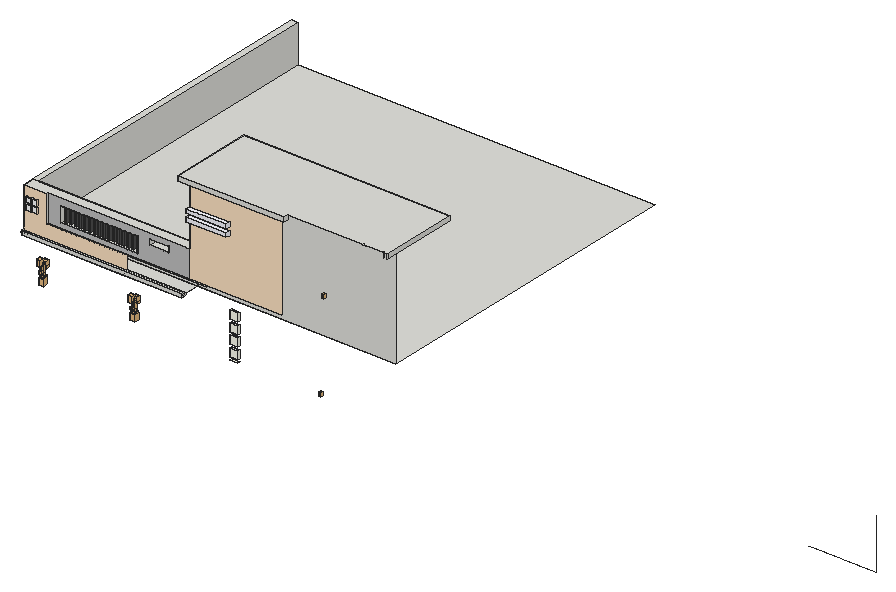
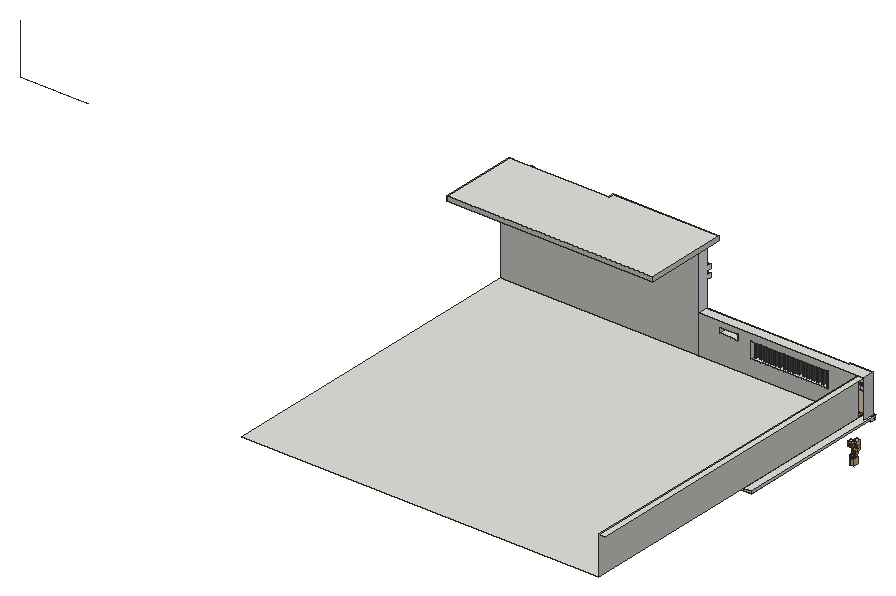
# SketchUp Ruby script. Lengths in inches.
U = 1.inch
M = Sketchup.active_model
def pt(a) = Geom::Point3d.new(a.map { |v| v * U })
def face(e, loops, mat)
  f = e.add_face(loops[0].map { |a| pt(a) })
  loops[1..].each { |l| e.add_face(l.map { |a| pt(a) }).erase! }
  f.material = f.back_material = mat if mat
  f
end
# faces: each face lists its corners as indices into pts; further lists are holes
def faces(e, pts, list, mat = nil) = list.each { |f| face(e, (f[0].is_a?(Array) ? f : [f]).map { |l| l.map { |i| pts[i] } }, mat) }
# xy, xz, yz: faces in a plane at the given z, y or x. An outline is a flat list of corners, or four numbers for a rectangle; further outlines are holes
def ring(l) = l.size == 4 ? [[l[0], l[1]], [l[2], l[1]], [l[2], l[3]], [l[0], l[3]]] : l.each_slice(2).to_a
def flat(e, list, mat, &to3) = list.each { |f| face(e, (f[0].is_a?(Array) ? f : [f]).map { |l| ring(l).map { |u, v| to3.(u, v) } }, mat) }
def xy(e, z, list, mat = nil) = flat(e, list, mat) { |x, y| [x, y, z] }
def xz(e, y, list, mat = nil) = flat(e, list, mat) { |x, z| [x, y, z] }
def yz(e, x, list, mat = nil) = flat(e, list, mat) { |y, z| [x, y, z] }
def lines(e, pts, list) = list.each { |a, b| e.add_line(pt(pts[a]), pt(pts[b])) }
# prism: a flat outline (further loops are holes) pulled along v
def prism(e, loops, v, mat = nil)
  f = face(e, loops, mat); d = Geom::Vector3d.new(v.map { |x| x * U })
  f.pushpull(f.normal.samedirection?(d) ? d.length : -d.length)
end
def box(e, o, s, mat = nil) = prism(e, [[o, [o[0] + s[0], o[1], o[2]], [o[0] + s[0], o[1] + s[1], o[2]], [o[0], o[1] + s[1], o[2]]]], [0, 0, s[2]], mat)
def at(x, y, z, deg = 0) = Geom::Transformation.translation(pt([x, y, z])) * Geom::Transformation.rotation(ORIGIN, Z_AXIS, deg.degrees)
def axes(o, x, y, z) = Geom::Transformation.new([*x, 0, *y, 0, *z, 0, *pt(o).to_a, 1])
def part(name) = M.definitions.add(name)
# library, detail: a bought-in or finely detailed component or shape, given as its bounding box
def library(name, o, s) = part(name).tap { |d| box(d.entities, o, s) }
def detail(e, o, s) = box(e.add_group.entities, o, s)
def put(e, d, t, mat = nil) = e.add_instance(d, t).tap { |i| i.material = mat if mat }
def group(e, t, mat = nil) = e.add_group.tap { |g| g.transformation = t; g.material = mat if mat }.entities
root = M.entities
M.materials.add("POT_TEXTURE_2").color = [160, 154, 144]
M.materials.add("[0012_Bisque]").color = [255, 228, 196]
M.materials.add("[0053_Ivory]").color = [255, 255, 240]
M.materials.add("[0117_GhostWhite]").color = [248, 248, 255]
M.materials.add("[0128_White]").color = [255, 255, 255]
M.materials.add("[0131_Silver]").color = [192, 192, 192]
M.materials.add("[0135_DarkGray]").color = [81, 81, 81]
M.materials.add("soil1").color = [68, 55, 47]
M.materials.add("wood_1").color = [140, 119, 94]
c1 = library("Group\#107",[-492.14,-508.4,-4.15],[433.72,431.71,567.03])
c2 = library("Lamp Wall Outdoor 94-02",[-1.89,-4.65,-3.17],[3.78,4.65,6.35])
c3 = library("Group\#106",[-385.21,-446.52,494.02],[160.93,321.12,1142.36])
c4 = library("Group\#81",[-447.02,-464.95,536.35],[343.73,346.24,39.39])
c5 = library("Group\#83",[-246.45,-349.05,558.47],[136.91,100.49,66.1])
c6 = library("Group\#103",[-293.78,-482.77,597.9],[158.75,112.78,159.87])
c7 = library("Group\#80",[-258.04,-282.68,604.05],[115.53,137.01,52.63])
c8 = library("Group\#88",[-304.79,-269.16,622.65],[82.06,111.89,102.57])
c9 = library("Group\#85",[-438.92,-265.61,702.3],[171.52,146.16,133.5])
c10 = library("Group\#97",[-295.03,-516.52,742.34],[68.71,141.75,78.67])
c11 = library("Group\#91",[-341.93,-403.49,744.8125],[64.83,96.32,132.15])
c12 = library("Group\#92",[-424,-312.27,817.53],[158.81,108.06,136.45])
c13 = library("Group\#95",[-388.93,-514.39,838.93],[89.79,77.73,82.08])
c14 = library("Group\#104",[-422.77,-235.4,843.61],[178.54,197.77,233.54])
c15 = library("Group\#98",[-498.98,-524.4,908.45],[120.83,107.95,112.98])
c16 = library("Group\#82",[-394.9,-448.99,911.74],[90.19,96.88,85.93])
c17 = library("Group\#96",[-409.02,-515.05,915.53],[69.62,77.27,65.47])
c18 = library("Group\#87",[-545.09,-386.51,922.3125],[300.25,219.65,227.33])
c19 = library("Group\#84",[-249.18,-250.59,980.93],[152.21,116.16,134.05])
c20 = library("Group\#90",[-244.55,-305.59,1009.46],[103.13,76.81,77.34])
c21 = library("Group\#89",[-292.14,-288.9,1281.79],[169.55,204.34,203.36])
c22 = library("Group\#94",[-568.91,-444.37,1285.4],[307.6,179.39,277.93])
c23 = library("Group\#101",[-321.08,-139.66,1308.49],[285.55,393.29,221.53])
c24 = library("Group\#105",[-292.81,-667.38,1418.14],[215.17,356.07,188.87])
c25 = library("Group\#93",[-357.04,-394.18,1447.05],[213.62,306.36,356.95])
c26 = library("Group\#100",[-548.25,-262.82,1459.54],[373.26,352.35,568])
c27 = library("Group\#102",[-387.74,-136.11,1470.07],[230,321.58,230.27])
c28 = library("Group\#86",[-264.68,-415.73,1484.11],[304.64,209.69,227.41])
c29 = library("Group\#99",[-278.4,-571.99,1530.91],[311.57,345.77,423.62])
xy(root,157.04,[[371.76,2122.39,386.07,2125.58]],"[0053_Ivory]")
xy(root,162.76,[[371.76,2122.39,386.07,2125.58]],"[0053_Ivory]")
xy(root,177.07,[[371.76,2122.39,386.07,2125.58]],"[0053_Ivory]")
xy(root,182.79,[[371.76,2122.39,386.07,2125.58]],"[0053_Ivory]")
xy(root,197.11,[[371.76,2122.39,386.07,2125.58]],"[0053_Ivory]")
xy(root,202.82,[[371.76,2122.39,386.07,2125.58]],"[0053_Ivory]")
xy(root,213,[[67.09,2396.39,119.53,2414.64]])
xy(root,217.14,[[371.76,2122.39,386.07,2125.58]],"[0053_Ivory]")
xy(root,219.25,[[185.8,2396.39,250.98,2410.14]])
xy(root,222.86,[[371.76,2122.39,386.07,2125.58]],"[0053_Ivory]")
xy(root,229.625,[[0,2117.95,185.58,2123.01],[185.58,2117.95,287.74,2123.01],[0,2123.01,287.74,2128.01]])
xy(root,233,[[0,2128.01,287.74,2396.39]])
xy(root,236.3125,[[0,2115.7,12.86,2117.95],[0,2117.95,12.86,2119.76],[12.86,2117.95,287.74,2123.01],[0,2119.76,12.86,2123.01],[0,2123.01,12.86,2396.39]])
xy(root,237.17,[[371.76,2122.39,386.07,2125.58]],"[0053_Ivory]")
xy(root,240,[[10.1875,2143.83,651.875,2725.58]])
xy(root,260.25,[[41.49,2123.01,329.67,2125.58]])
xy(root,264.46,[[127.75,2130.89,132.0625,2137.87]])
xy(root,265.71,[[179.2,2130.89,183.51,2137.87]])
xy(root,265.96,[[162.05,2130.89,166.36,2137.87]])
xy(root,266.09,[[136.32,2130.89,140.64,2137.87]])
xy(root,266.15,[[144.9,2130.89,149.21,2137.87],[170.625,2130.89,174.9375,2137.87]])
xy(root,267.53,[[67.72,2130.89,72.04,2137.87]])
xy(root,267.78,[[84.875,2130.89,89.1875,2137.87]])
xy(root,267.9,[[[65.14,2125.58,202.96,2143.83],[76.3,2130.89,80.61,2137.87],[93.45,2130.89,97.76,2137.87],[102.02,2130.89,106.34,2137.87],[110.6,2130.89,114.91,2137.87],[119.17,2130.89,123.49,2137.87],[153.47,2130.89,157.79,2137.87],[187.77,2130.89,192.09,2137.87],[196.35,2130.89,200.66,2137.87]]])
xy(root,270.92,[[5.13,2121.45,14.32,2123.01],[15.88,2121.45,25.07,2123.01]],"[0012_Bisque]")
xy(root,280.11,[[5.13,2121.45,14.32,2123.01],[15.88,2121.45,25.07,2123.01]],"[0012_Bisque]")
xy(root,282.8,[[5.07,2121.45,14.26,2123.01],[15.88,2121.45,25.07,2123.01]],"[0012_Bisque]")
xy(root,289.15,[[225.61,2125.58,259.17,2143.83]])
xy(root,291.98,[[15.88,2121.45,25.07,2123.01]],"[0012_Bisque]")
xy(root,291.98,[[5.07,2121.45,14.26,2123.01]],"[0128_White]")
xy(root,296.71,[[[65.14,2125.58,202.96,2143.83],[67.72,2130.89,72.04,2137.87],[76.3,2130.89,80.61,2137.87],[84.875,2130.89,89.1875,2137.87],[93.45,2130.89,97.76,2137.87],[102.02,2130.89,106.34,2137.87],[110.6,2130.89,114.91,2137.87],[119.17,2130.89,123.49,2137.87],[127.75,2130.89,132.0625,2137.87],[136.32,2130.89,140.64,2137.87],[144.9,2130.89,149.21,2137.87],[153.47,2130.89,157.79,2137.87],[162.05,2130.89,166.36,2137.87],[170.625,2130.89,174.9375,2137.87],[179.2,2130.89,183.51,2137.87],[187.77,2130.89,192.09,2137.87],[196.35,2130.89,200.66,2137.87]]])
xy(root,298.97,[[225.61,2125.58,259.17,2143.83]])
xy(root,308.3125,[[0,2123.01,41.49,2123.01,41.49,2125.58,295.9,2125.58,295.9,2143.83,0,2143.83],[0,2143.83,10.1875,2725.58]])
xy(root,354.72,[[295.9,2118.58,367.78,2125.58]],"[0012_Bisque]")
xy(root,362.04,[[295.9,2118.58,367.78,2125.58]],"[0117_GhostWhite]")
xy(root,368.47,[[295.9,2118.58,367.78,2125.58]],"[0012_Bisque]")
xy(root,375.79,[[295.9,2118.58,367.78,2125.58]],"[0117_GhostWhite]")
xy(root,416.5,[[282.34,2115.7,282.34,2264.76,651.875,2264.76,651.875,2143.83,295.9,2143.83,295.9,2125.58,461.86,2125.58,461.86,2115.7]])
xy(root,425.125,[[282.34,2115.7,472.61,2115.7,472.61,2125.58,651.875,2125.58,651.875,2264.76,282.34,2264.76],[608.45,2124.78,613.45,2125.58],[645.875,2124.78,651.875,2125.58]])
xz(root,2115.7,[[282.34,416.5,461.86,416.5,461.86,417.125,472.61,417.125,472.61,425.125,282.34,425.125]])
xz(root,2117.95,[[0,229.625,287.74,236.3125]])
xz(root,2118.58,[[295.9,354.72,367.78,362.04],[295.9,368.47,367.78,375.79]],"[0117_GhostWhite]")
xz(root,2121.45,[[5.13,270.92,14.32,280.11],[15.88,270.92,25.07,280.11],[5.07,282.8,14.26,291.98],[15.88,282.8,25.07,291.98]],"[0128_White]")
xz(root,2122.39,[[371.76,162.76,386.07,177.07],[371.76,182.79,386.07,197.11],[371.76,202.82,386.07,217.14],[371.76,222.86,386.07,237.17]],"[0053_Ivory]")
xz(root,2123.01,[[185.58,229.625,287.74,233],[185.58,233,287.74,236.3125]])
xz(root,2123.01,[[[0,236.3125,185.58,236.3125,185.58,260.25,41.49,260.25,41.49,308.3125,0,308.3125],[5.07,282.8,14.26,291.98],[15.88,282.8,25.07,291.98],[15.88,270.92,25.07,280.11],[5.13,270.92,14.32,280.11]]],"[0012_Bisque]")
xz(root,2125.58,[[295.9,416.5,461.86,417.125]])
xz(root,2125.58,[[295.9,260.25,461.86,260.25,461.86,416.5,295.9,416.5,295.9,375.79,367.78,375.79,367.78,368.47,295.9,368.47,295.9,362.04,367.78,362.04,367.78,354.72,295.9,354.72]],"[0012_Bisque]")
xz(root,2125.58,[[371.76,162.76,386.07,177.07],[371.76,182.79,386.07,197.11],[371.76,202.82,386.07,217.14],[371.76,222.86,386.07,237.17],[[41.49,260.25,295.9,308.3125],[65.14,267.9,202.96,296.71],[225.61,289.15,259.17,298.97]]],"[0131_Silver]")
xz(root,2128.01,[[0,229.625,185.58,233],[185.58,229.625,287.74,233]])
xz(root,2130.89,[[127.75,264.46,132.0625,296.71],[179.2,265.71,183.51,296.71],[162.05,265.96,166.36,296.71],[136.32,266.09,140.64,296.71],[144.9,266.15,149.21,296.71],
  [170.625,266.15,174.9375,296.71],[67.72,267.53,72.04,296.71],[84.875,267.78,89.1875,296.71],[76.3,267.9,80.61,296.71],[93.45,267.9,97.76,296.71],
  [102.02,267.9,106.34,296.71],[110.6,267.9,114.91,296.71],[119.17,267.9,123.49,296.71],[153.47,267.9,157.79,296.71],[187.77,267.9,192.09,296.71],
  [196.35,267.9,200.66,296.71]],"[0135_DarkGray]")
xz(root,2137.87,[[127.75,264.46,132.0625,296.71],[179.2,265.71,183.51,296.71],[162.05,265.96,166.36,296.71],[136.32,266.09,140.64,296.71],[144.9,266.15,149.21,296.71],
  [170.625,266.15,174.9375,296.71],[67.72,267.53,72.04,296.71],[84.875,267.78,89.1875,296.71],[76.3,267.9,80.61,296.71],[93.45,267.9,97.76,296.71],
  [102.02,267.9,106.34,296.71],[110.6,267.9,114.91,296.71],[119.17,267.9,123.49,296.71],[153.47,267.9,157.79,296.71],[187.77,267.9,192.09,296.71],
  [196.35,267.9,200.66,296.71]],"[0135_DarkGray]")
xz(root,2143.83,[[[10.1875,240,295.9,308.3125],[65.14,267.9,202.96,296.71],[225.61,289.15,259.17,298.97]],[295.9,240,651.875,416.5],[295.9,416.5,651.875,417.125]])
xz(root,2264.76,[[282.34,416.5,651.875,425.125]])
xz(root,2396.39,[[0,233,12.86,236.3125]])
yz(root,0,[[2117.95,229.625,2119.76,236.3125],[2119.76,229.625,2119.76,236.3125,2396.39,236.3125,2396.39,233,2128.01,233,2128.01,229.625],[2123.01,240,2143.83,308.3125]])
yz(root,5.07,[[2121.45,282.8,2123.01,291.98]],"[0128_White]")
yz(root,5.13,[[2121.45,270.92,2123.01,280.11]],"[0128_White]")
yz(root,10.1875,[[2143.83,240,2725.58,308.3125]])
yz(root,14.26,[[2121.45,282.8,2123.01,291.98]],"[0012_Bisque]")
yz(root,14.32,[[2121.45,270.92,2123.01,280.11]],"[0012_Bisque]")
yz(root,15.88,[[2121.45,270.92,2123.01,280.11],[2121.45,282.8,2123.01,291.98]],"[0128_White]")
yz(root,25.07,[[2121.45,270.92,2123.01,280.11],[2121.45,282.8,2123.01,291.98]],"[0012_Bisque]")
yz(root,41.49,[[2123.01,260.25,2125.58,308.3125]])
yz(root,65.14,[[2125.58,267.9,2143.83,296.71]])
yz(root,67.72,[[2130.89,267.53,2137.87,296.71]],"[0135_DarkGray]")
yz(root,72.04,[[2130.89,267.53,2137.87,296.71]],"[0135_DarkGray]")
yz(root,76.3,[[2130.89,267.9,2137.87,296.71]],"[0135_DarkGray]")
yz(root,80.61,[[2130.89,267.9,2137.87,296.71]],"[0135_DarkGray]")
yz(root,84.875,[[2130.89,267.78,2137.87,296.71]],"[0135_DarkGray]")
yz(root,89.1875,[[2130.89,267.78,2137.87,296.71]],"[0135_DarkGray]")
yz(root,93.45,[[2130.89,267.9,2137.87,296.71]],"[0135_DarkGray]")
yz(root,97.76,[[2130.89,267.9,2137.87,296.71]],"[0135_DarkGray]")
yz(root,102.02,[[2130.89,267.9,2137.87,296.71]],"[0135_DarkGray]")
yz(root,106.34,[[2130.89,267.9,2137.87,296.71]],"[0135_DarkGray]")
yz(root,110.6,[[2130.89,267.9,2137.87,296.71]],"[0135_DarkGray]")
yz(root,114.91,[[2130.89,267.9,2137.87,296.71]],"[0135_DarkGray]")
yz(root,119.17,[[2130.89,267.9,2137.87,296.71]],"[0135_DarkGray]")
yz(root,123.49,[[2130.89,267.9,2137.87,296.71]],"[0135_DarkGray]")
yz(root,127.75,[[2130.89,264.46,2137.87,296.71]],"[0135_DarkGray]")
yz(root,132.0625,[[2130.89,264.46,2137.87,296.71]],"[0135_DarkGray]")
yz(root,136.32,[[2130.89,266.09,2137.87,296.71]],"[0135_DarkGray]")
yz(root,140.64,[[2130.89,266.09,2137.87,296.71]],"[0135_DarkGray]")
yz(root,144.9,[[2130.89,266.15,2137.87,296.71]],"[0135_DarkGray]")
yz(root,149.21,[[2130.89,266.15,2137.87,296.71]],"[0135_DarkGray]")
yz(root,153.47,[[2130.89,267.9,2137.87,296.71]],"[0135_DarkGray]")
yz(root,157.79,[[2130.89,267.9,2137.87,296.71]],"[0135_DarkGray]")
yz(root,162.05,[[2130.89,265.96,2137.87,296.71]],"[0135_DarkGray]")
yz(root,166.36,[[2130.89,265.96,2137.87,296.71]],"[0135_DarkGray]")
yz(root,170.625,[[2130.89,266.15,2137.87,296.71]],"[0135_DarkGray]")
yz(root,174.9375,[[2130.89,266.15,2137.87,296.71]],"[0135_DarkGray]")
yz(root,179.2,[[2130.89,265.71,2137.87,296.71]],"[0135_DarkGray]")
yz(root,183.51,[[2130.89,265.71,2137.87,296.71]],"[0135_DarkGray]")
yz(root,187.77,[[2130.89,267.9,2137.87,296.71]],"[0135_DarkGray]")
yz(root,192.09,[[2130.89,267.9,2137.87,296.71]],"[0135_DarkGray]")
yz(root,196.35,[[2130.89,267.9,2137.87,296.71]],"[0135_DarkGray]")
yz(root,200.66,[[2130.89,267.9,2137.87,296.71]],"[0135_DarkGray]")
yz(root,202.96,[[2125.58,267.9,2143.83,296.71]])
yz(root,225.61,[[2125.58,289.15,2143.83,298.97]])
yz(root,259.17,[[2125.58,289.15,2143.83,298.97]])
yz(root,282.34,[[2115.7,416.5,2264.76,425.125]])
yz(root,287.74,[[2117.95,229.625,2123.01,233],[2123.01,229.625,2128.01,233],[2117.95,233,2123.01,236.3125]])
yz(root,295.9,[[2125.58,416.5,2143.83,417.125]])
yz(root,295.9,[[2125.58,308.3125,2125.58,354.72,2118.58,354.72,2118.58,362.04,2125.58,362.04,2125.58,368.47,2118.58,368.47,2118.58,375.79,2125.58,375.79,2125.58,416.5,2143.83,416.5,2143.83,308.3125]],"[0117_GhostWhite]")
yz(root,367.78,[[2118.58,354.72,2125.58,362.04],[2118.58,368.47,2125.58,375.79]],"[0117_GhostWhite]")
yz(root,371.76,[[2122.39,162.76,2125.58,177.07],[2122.39,182.79,2125.58,197.11],[2122.39,202.82,2125.58,217.14],[2122.39,222.86,2125.58,237.17]],"[0053_Ivory]")
yz(root,386.07,[[2122.39,162.76,2125.58,177.07],[2122.39,182.79,2125.58,197.11],[2122.39,202.82,2125.58,217.14],[2122.39,222.86,2125.58,237.17]],"[0053_Ivory]")
yz(root,461.86,[[2115.7,416.5,2125.58,417.125]])
yz(root,472.61,[[2115.7,417.125,2125.58,425.125]])
yz(root,645.875,[[2124.78,417.125,2125.58,425.125]])
yz(root,651.875,[[2143.83,416.5,2264.76,416.5,2264.76,425.125,2125.58,425.125,2125.58,417.125,2143.83,417.125],[2124.78,417.125,2125.58,425.125]])
p = [[295.9,2125.58,240],[295.9,2143.83,240],[0,2123.01,233],[185.58,2123.01,233],[185.58,2117.95,233],[22.06,2137.24,154.04],
  [22.06,2137.26,154.04],[22.04,2137.26,154.04],[186.04,2137.26,154.04],[186.02,2137.26,154.04],[186.04,2137.24,154.04],[1422.97,2107.36,233.67],
  [1544.53,2107.36,233.67],[1544.53,2107.36,325.35]]
lines(root,p,[[0,1],[2,3],[3,4],[5,6],[6,7],[7,5],[8,9],[10,8],[9,10],[11,12],[12,13]])
put(root,c1,axes([22.06,2137.24,154.04],[0,0.0198,0],[-0.0198,0,0],[0,0,0.0198]),"POT_TEXTURE_2")
put(root,c1,axes([186.04,2137.24,154.04],[0,0.0198,0],[-0.0198,0,0],[0,0,0.0198]),"POT_TEXTURE_2")
put(root,c2,at(534.21,2125.58,159.29))
put(root,c3,axes([22.06,2137.24,154.04],[0,0.0198,0],[-0.0198,0,0],[0,0,0.0198]),"wood_1")
put(root,c3,axes([186.04,2137.24,154.04],[0,0.0198,0],[-0.0198,0,0],[0,0,0.0198]),"wood_1")
put(root,c4,axes([22.06,2137.24,154.04],[0,0.0198,0],[-0.0198,0,0],[0,0,0.0198]),"soil1")
put(root,c4,axes([186.04,2137.24,154.04],[0,0.0198,0],[-0.0198,0,0],[0,0,0.0198]),"soil1")
put(root,c5,axes([22.06,2137.24,154.04],[0,0.0198,0],[-0.0198,0,0],[0,0,0.0198]))
put(root,c5,axes([186.04,2137.24,154.04],[0,0.0198,0],[-0.0198,0,0],[0,0,0.0198]))
put(root,c6,axes([22.06,2137.24,154.04],[0,0.0198,0],[-0.0198,0,0],[0,0,0.0198]))
put(root,c6,axes([186.04,2137.24,154.04],[0,0.0198,0],[-0.0198,0,0],[0,0,0.0198]))
put(root,c7,axes([22.06,2137.24,154.04],[0,0.0198,0],[-0.0198,0,0],[0,0,0.0198]))
put(root,c7,axes([186.04,2137.24,154.04],[0,0.0198,0],[-0.0198,0,0],[0,0,0.0198]))
put(root,c8,axes([22.06,2137.24,154.04],[0,0.0198,0],[-0.0198,0,0],[0,0,0.0198]))
put(root,c8,axes([186.04,2137.24,154.04],[0,0.0198,0],[-0.0198,0,0],[0,0,0.0198]))
put(root,c9,axes([22.06,2137.24,154.04],[0,0.0198,0],[-0.0198,0,0],[0,0,0.0198]))
put(root,c9,axes([186.04,2137.24,154.04],[0,0.0198,0],[-0.0198,0,0],[0,0,0.0198]))
put(root,c10,axes([22.06,2137.24,154.04],[0,0.0198,0],[-0.0198,0,0],[0,0,0.0198]))
put(root,c10,axes([186.04,2137.24,154.04],[0,0.0198,0],[-0.0198,0,0],[0,0,0.0198]))
put(root,c11,axes([22.06,2137.24,154.04],[0,0.0198,0],[-0.0198,0,0],[0,0,0.0198]))
put(root,c11,axes([186.04,2137.24,154.04],[0,0.0198,0],[-0.0198,0,0],[0,0,0.0198]))
put(root,c12,axes([22.06,2137.24,154.04],[0,0.0198,0],[-0.0198,0,0],[0,0,0.0198]))
put(root,c12,axes([186.04,2137.24,154.04],[0,0.0198,0],[-0.0198,0,0],[0,0,0.0198]))
put(root,c13,axes([22.06,2137.24,154.04],[0,0.0198,0],[-0.0198,0,0],[0,0,0.0198]))
put(root,c13,axes([186.04,2137.24,154.04],[0,0.0198,0],[-0.0198,0,0],[0,0,0.0198]))
put(root,c14,axes([22.06,2137.24,154.04],[0,0.0198,0],[-0.0198,0,0],[0,0,0.0198]))
put(root,c14,axes([186.04,2137.24,154.04],[0,0.0198,0],[-0.0198,0,0],[0,0,0.0198]))
put(root,c15,axes([22.06,2137.24,154.04],[0,0.0198,0],[-0.0198,0,0],[0,0,0.0198]))
put(root,c15,axes([186.04,2137.24,154.04],[0,0.0198,0],[-0.0198,0,0],[0,0,0.0198]))
put(root,c16,axes([22.06,2137.24,154.04],[0,0.0198,0],[-0.0198,0,0],[0,0,0.0198]))
put(root,c16,axes([186.04,2137.24,154.04],[0,0.0198,0],[-0.0198,0,0],[0,0,0.0198]))
put(root,c17,axes([22.06,2137.24,154.04],[0,0.0198,0],[-0.0198,0,0],[0,0,0.0198]))
put(root,c17,axes([186.04,2137.24,154.04],[0,0.0198,0],[-0.0198,0,0],[0,0,0.0198]))
put(root,c18,axes([22.06,2137.24,154.04],[0,0.0198,0],[-0.0198,0,0],[0,0,0.0198]))
put(root,c18,axes([186.04,2137.24,154.04],[0,0.0198,0],[-0.0198,0,0],[0,0,0.0198]))
put(root,c19,axes([22.06,2137.24,154.04],[0,0.0198,0],[-0.0198,0,0],[0,0,0.0198]))
put(root,c19,axes([186.04,2137.24,154.04],[0,0.0198,0],[-0.0198,0,0],[0,0,0.0198]))
put(root,c20,axes([22.06,2137.24,154.04],[0,0.0198,0],[-0.0198,0,0],[0,0,0.0198]))
put(root,c20,axes([186.04,2137.24,154.04],[0,0.0198,0],[-0.0198,0,0],[0,0,0.0198]))
put(root,c21,axes([22.06,2137.24,154.04],[0,0.0198,0],[-0.0198,0,0],[0,0,0.0198]))
put(root,c21,axes([186.04,2137.24,154.04],[0,0.0198,0],[-0.0198,0,0],[0,0,0.0198]))
put(root,c22,axes([22.06,2137.24,154.04],[0,0.0198,0],[-0.0198,0,0],[0,0,0.0198]))
put(root,c22,axes([186.04,2137.24,154.04],[0,0.0198,0],[-0.0198,0,0],[0,0,0.0198]))
put(root,c23,axes([22.06,2137.24,154.04],[0,0.0198,0],[-0.0198,0,0],[0,0,0.0198]))
put(root,c23,axes([186.04,2137.24,154.04],[0,0.0198,0],[-0.0198,0,0],[0,0,0.0198]))
put(root,c24,axes([22.06,2137.24,154.04],[0,0.0198,0],[-0.0198,0,0],[0,0,0.0198]))
put(root,c24,axes([186.04,2137.24,154.04],[0,0.0198,0],[-0.0198,0,0],[0,0,0.0198]))
put(root,c25,axes([22.06,2137.24,154.04],[0,0.0198,0],[-0.0198,0,0],[0,0,0.0198]))
put(root,c25,axes([186.04,2137.24,154.04],[0,0.0198,0],[-0.0198,0,0],[0,0,0.0198]))
put(root,c26,axes([22.06,2137.24,154.04],[0,0.0198,0],[-0.0198,0,0],[0,0,0.0198]))
put(root,c26,axes([186.04,2137.24,154.04],[0,0.0198,0],[-0.0198,0,0],[0,0,0.0198]))
put(root,c27,axes([22.06,2137.24,154.04],[0,0.0198,0],[-0.0198,0,0],[0,0,0.0198]))
put(root,c27,axes([186.04,2137.24,154.04],[0,0.0198,0],[-0.0198,0,0],[0,0,0.0198]))
put(root,c28,axes([22.06,2137.24,154.04],[0,0.0198,0],[-0.0198,0,0],[0,0,0.0198]))
put(root,c28,axes([186.04,2137.24,154.04],[0,0.0198,0],[-0.0198,0,0],[0,0,0.0198]))
put(root,c29,axes([22.06,2137.24,154.04],[0,0.0198,0],[-0.0198,0,0],[0,0,0.0198]))
put(root,c29,axes([186.04,2137.24,154.04],[0,0.0198,0],[-0.0198,0,0],[0,0,0.0198]))
put(root,c2,at(539.78,2125.58,318.66))
